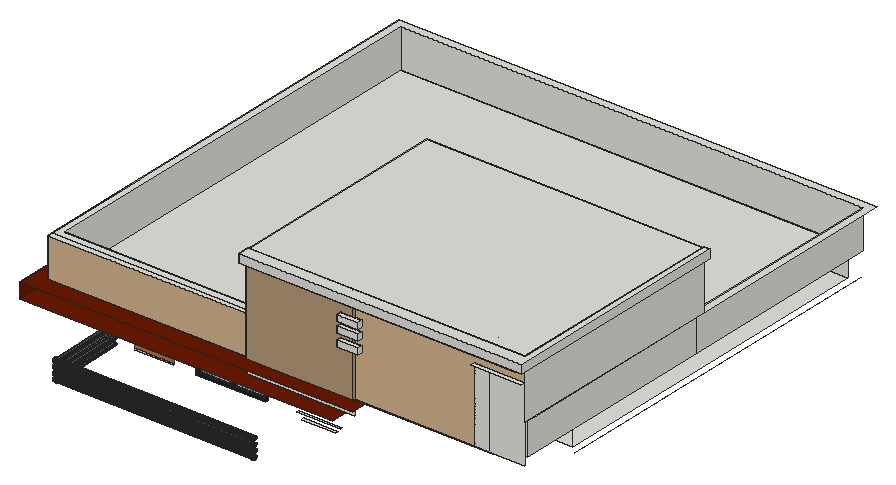
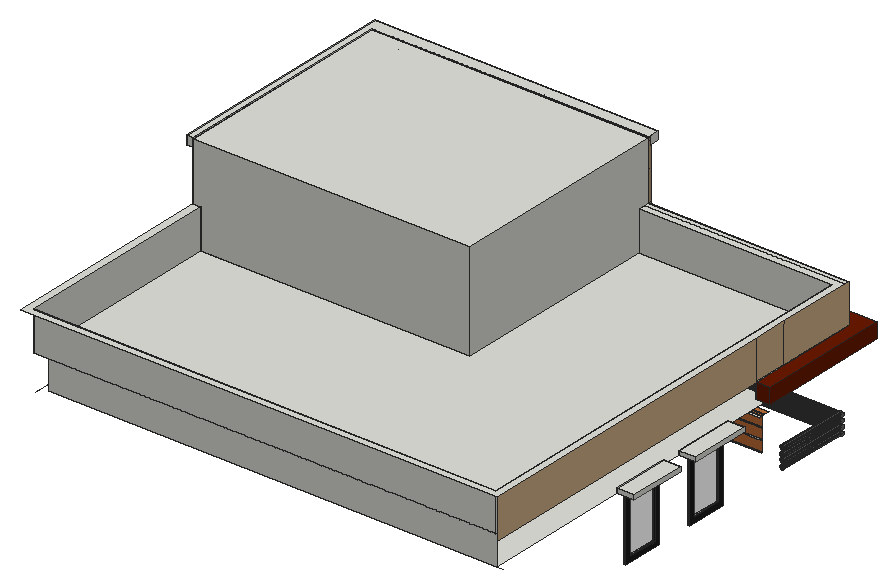
# SketchUp Ruby script. Lengths in inches.
U = 1.inch
M = Sketchup.active_model
def pt(a) = Geom::Point3d.new(a.map { |v| v * U })
def face(e, loops, mat)
  f = e.add_face(loops[0].map { |a| pt(a) })
  loops[1..].each { |l| e.add_face(l.map { |a| pt(a) }).erase! }
  f.material = f.back_material = mat if mat
  f
end
# faces: each face lists its corners as indices into pts; further lists are holes
def faces(e, pts, list, mat = nil) = list.each { |f| face(e, (f[0].is_a?(Array) ? f : [f]).map { |l| l.map { |i| pts[i] } }, mat) }
# xy, xz, yz: faces in a plane at the given z, y or x. An outline is a flat list of corners, or four numbers for a rectangle; further outlines are holes
def ring(l) = l.size == 4 ? [[l[0], l[1]], [l[2], l[1]], [l[2], l[3]], [l[0], l[3]]] : l.each_slice(2).to_a
def flat(e, list, mat, &to3) = list.each { |f| face(e, (f[0].is_a?(Array) ? f : [f]).map { |l| ring(l).map { |u, v| to3.(u, v) } }, mat) }
def xy(e, z, list, mat = nil) = flat(e, list, mat) { |x, y| [x, y, z] }
def xz(e, y, list, mat = nil) = flat(e, list, mat) { |x, z| [x, y, z] }
def yz(e, x, list, mat = nil) = flat(e, list, mat) { |y, z| [x, y, z] }
def lines(e, pts, list) = list.each { |a, b| e.add_line(pt(pts[a]), pt(pts[b])) }
# prism: a flat outline (further loops are holes) pulled along v
def prism(e, loops, v, mat = nil)
  f = face(e, loops, mat); d = Geom::Vector3d.new(v.map { |x| x * U })
  f.pushpull(f.normal.samedirection?(d) ? d.length : -d.length)
end
def box(e, o, s, mat = nil) = prism(e, [[o, [o[0] + s[0], o[1], o[2]], [o[0] + s[0], o[1] + s[1], o[2]], [o[0], o[1] + s[1], o[2]]]], [0, 0, s[2]], mat)
def at(x, y, z, deg = 0) = Geom::Transformation.translation(pt([x, y, z])) * Geom::Transformation.rotation(ORIGIN, Z_AXIS, deg.degrees)
def axes(o, x, y, z) = Geom::Transformation.new([*x, 0, *y, 0, *z, 0, *pt(o).to_a, 1])
def part(name) = M.definitions.add(name)
# library, detail: a bought-in or finely detailed component or shape, given as its bounding box
def library(name, o, s) = part(name).tap { |d| box(d.entities, o, s) }
def detail(e, o, s) = box(e.add_group.entities, o, s)
def put(e, d, t, mat = nil) = e.add_instance(d, t).tap { |i| i.material = mat if mat }
def group(e, t, mat = nil) = e.add_group.tap { |g| g.transformation = t; g.material = mat if mat }.entities
root = M.entities
M.materials.add("[0035_Tan]").color = [181, 154, 120]
M.materials.add("[0035_Tan]1").color = [210, 180, 140]
M.materials.add("[0134_DimGray]").color = [105, 105, 105]
M.materials.add("[Color B07]").color = [107, 26, 0]
M.materials.add("[Color M08]").color = [30, 30, 30]
M.materials.add("[Translucent Glass Blue]").color = [61, 91, 145]
M.materials["[Translucent Glass Blue]"].alpha = 0.5
M.materials.add("[Translucent Glass Gray]").color = [128, 128, 128]
M.materials["[Translucent Glass Gray]"].alpha = 0.5
M.materials.add("[Wood Veneer 01]").color = [191, 111, 58]
prism(root,[[[13.875,208.16,859.6875],[13.875,283.03,859.6875],[34.875,283.03,859.6875],[34.875,273.28,859.6875],[34.875,208.16,859.6875]]],[0,0,5.375])
prism(root,[[[34.875,378.1,859.6875],[34.875,312.97,859.6875],[34.875,306.78,859.6875],[13.875,306.78,859.6875],[13.875,378.1,859.6875]]],[0,0,5.375])
xy(root,777.125,[[141.33,116.9375,227.02,119.9375]])
xy(root,777.36,[[31.875,219.0625,34.875,270.0625]])
xy(root,777.36,[[31.875,317.1875,34.875,368.1875]],"[Color M08]")
xy(root,780.125,[[144.33,116.9375,184.18,119.9375],[187.18,116.9375,224.02,119.9375]],"[Color M08]")
xy(root,783.36,[[31.875,225.0625,34.875,264.0625],[31.875,323.1875,34.875,362.1875]],"[Color M08]")
xy(root,819,[[65.96,116.9375,113.96,119.9375]])
xy(root,819,[[65.96,113.9375,113.96,116.9375]],"[Wood Veneer 01]")
xy(root,825,[[59.96,113.9375,119.96,119.9375]],"[Wood Veneer 01]")
xy(root,834.8125,[[144.33,116.9375,184.18,119.9375],[187.18,116.9375,224.02,119.9375]],"[Color M08]")
xy(root,837.8125,[[141.33,116.9375,227.02,119.9375]],"[Color M08]")
xy(root,844.6875,[[350.38,17.9375,392.07,20.9375]])
xy(root,850.6875,[[344.38,17.9375,398.07,20.9375]])
xy(root,851.18,[[31.875,225.0625,34.875,264.0625],[31.875,323.1875,34.875,362.1875]],"[Color M08]")
xy(root,852,[[43.875,128.9375,595.125,552.98]])
xy(root,857.18,[[31.875,219.0625,34.875,270.0625],[31.875,317.1875,34.875,368.1875]],"[Color M08]")
xy(root,869.45,[[18.22,0,18.22,164.4375,35.6,164.4375,35.6,26.9375,282.125,26.9375,282.125,20.9375,402.53,20.9375,402.53,0]],"[Color B07]")
xy(root,882.89,[[35.6,26.9375,35.6,119.9375,578.6875,119.9375,578.6875,35.9375,282.125,35.9375,282.125,26.9375],[282.125,26.9375,578.6875,35.9375]])
xy(root,888,[[282.125,17.9375,413.18,20.9375],[35.6,20.9375,578.6875,26.9375],[44.6,35.9375,282.125,35.9375,282.125,296,614,296,614,552.98,44.6,552.98],[282.125,35.9375,614,296],[34.875,119.9375,35.6,128.9375],
  [34.875,128.9375,35.6,164.4375]])
xy(root,888,[[18.22,0,427.625,0,427.625,20.9375,413.18,20.9375,413.18,17.9375,282.125,17.9375,282.125,20.9375,35.6,20.9375,35.6,119.9375,34.875,119.9375,34.875,164.4375,18.22,164.4375]],"[Color B07]")
xy(root,936,[[35.6,20.9375,282.125,26.9375],[35.6,26.9375,282.125,26.9375,282.125,35.9375,44.6,35.9375,44.6,552.98,614,552.98,614,296,623,296,623,561.98,34.875,561.98,34.875,164.4375,35.6,164.4375],[282.125,26.9375,578.6875,35.9375],[578.6875,26.9375,623,35.9375],[614,35.9375,623,296]])
xy(root,944.65,[[398.24,11.9375,424.12,17.9375]])
xy(root,952.1,[[398.24,11.9375,424.12,17.9375]])
xy(root,959.84,[[398.24,11.9375,424.12,17.9375]])
xy(root,967.29,[[398.24,11.9375,424.12,17.9375]])
xy(root,972.59,[[398.24,11.9375,424.12,17.9375]])
xy(root,980,[[561.08,14.9375,623,20.9375]])
xy(root,980.04,[[398.24,11.9375,424.12,17.9375]])
xy(root,998.73,[[282.125,5.9375,282.125,17.9375,413.18,17.9375,413.18,20.9375,623,20.9375,623,5.9375],[623,5.9375,630.81,296]])
xy(root,1008,[[282.125,20.9375,623,296]])
xy(root,1009.125,[[282.125,5.9375,630.81,5.9375,630.81,296,623,296,623,20.9375,282.125,20.9375]])
xz(root,5.9375,[[282.125,998.73,630.81,1009.125]])
xz(root,11.9375,[[398.24,944.65,424.12,952.1],[398.24,959.84,424.12,967.29],[398.24,972.59,424.12,980.04]])
xz(root,17.9375,[[398.24,944.65,413.18,952.1],[413.18,944.65,424.12,952.1],[398.24,959.84,413.18,967.29],[413.18,959.84,424.12,967.29],[398.24,972.59,413.18,980.04],
  [413.18,972.59,424.12,980.04]])
xz(root,17.9375,[[282.125,888,413.18,888,413.18,944.65,398.24,944.65,398.24,952.1,413.18,952.1,413.18,959.84,398.24,959.84,398.24,967.29,413.18,967.29,413.18,972.59,398.24,972.59,398.24,980.04,413.18,980.04,413.18,998.73,282.125,998.73]],"[0035_Tan]")
xz(root,20.9375,[[282.125,869.45,413.18,888],[282.125,888,413.18,1008],[561.08,888,578.6875,980],[578.6875,888,623,980],[413.18,998.73,623,1008],
  [282.125,1008,623,1009.125]])
xz(root,20.9375,[[35.6,888,282.125,936],[413.18,888,561.08,888,561.08,980,623,980,623,998.73,413.18,998.73]],"[0035_Tan]1")
xz(root,26.9375,[[35.6,882.89,578.6875,888]])
xz(root,26.9375,[[35.6,869.45,282.125,882.89]],"[Color B07]")
xz(root,35.9375,[[44.6,888,282.125,936],[282.125,888,578.6875,936],[578.6875,888,614,936]])
xz(root,116.9375,[[65.96,778.55,113.96,779.87],[65.96,792.23,113.96,793.55],[65.96,805.92,113.96,807.24]])
xz(root,116.9375,[[[141.33,777.125,227.02,837.8125],[144.33,780.125,184.18,834.8125],[187.18,780.125,224.02,834.8125]]],"[Color M08]")
xz(root,116.9375,[[65.96,779.87,113.96,792.23],[65.96,793.55,113.96,805.92],[65.96,807.24,113.96,819]],"[Wood Veneer 01]")
xz(root,119.9375,[[[141.33,777.125,227.02,837.8125],[144.33,780.125,184.18,834.8125],[187.18,780.125,224.02,834.8125]],[34.875,852,35.6,882.89],[34.875,882.89,35.6,888]])
xz(root,119.9375,[[144.33,780.125,184.18,834.8125],[187.18,780.125,224.02,834.8125]],"[Translucent Glass Blue]")
xz(root,164.4375,[[34.875,888,35.6,936]])
xz(root,164.4375,[[18.22,869.45,35.6,888]],"[Color B07]")
xz(root,219.0625,[[31.875,777.36,34.875,857.18]],"[Color M08]")
xz(root,225.0625,[[31.875,783.36,34.875,851.18]],"[Color M08]")
xz(root,264.0625,[[31.875,783.36,34.875,851.18]],"[Color M08]")
xz(root,270.0625,[[31.875,777.36,34.875,857.18]],"[Color M08]")
xz(root,296,[[282.125,888,282.125,1008,623,1008,623,936,614,936,614,888],[623,998.73,630.81,1009.125]])
xz(root,317.1875,[[31.875,777.36,34.875,857.18]],"[Color M08]")
xz(root,323.1875,[[31.875,783.36,34.875,851.18]],"[Color M08]")
xz(root,362.1875,[[31.875,783.36,34.875,851.18]],"[Color M08]")
xz(root,368.1875,[[31.875,777.36,34.875,857.18]],"[Color M08]")
xz(root,552.98,[[43.875,852,595.125,888],[44.6,888,614,936]])
yz(root,18.22,[[0,869.45,164.4375,888]],"[Color B07]")
yz(root,31.875,[[[219.0625,777.36,270.0625,857.18],[225.0625,783.36,264.0625,851.18]],[[317.1875,777.36,368.1875,857.18],[323.1875,783.36,362.1875,851.18]]],"[Color M08]")
yz(root,34.875,[[[219.0625,777.36,270.0625,857.18],[225.0625,783.36,264.0625,851.18]],[[317.1875,777.36,368.1875,857.18],[323.1875,783.36,362.1875,851.18]]])
yz(root,34.875,[[164.4375,888,561.98,936]],"[0035_Tan]1")
yz(root,34.875,[[31.46,770.43,30.85,770.51,30.27,770.75,29.78,771.125,29.4,771.62,29.17,772.19,29.09,772.81,29.17,773.42,29.4,773.99,29.78,774.48,30.27,774.86,30.85,775.1,31.46,775.18,32.08,775.1,32.65,774.86,33.14,774.48,33.52,773.99,33.76,773.42,33.84,772.81,33.76,772.19,33.52,771.62,33.14,771.125,32.65,770.75,32.08,770.51],[31.46,777.49,30.85,777.57,30.27,777.8125,29.78,778.1875,29.4,778.68,29.17,779.25,29.09,779.87,29.17,780.48,29.4,781.06,29.78,781.55,30.27,781.92,30.85,782.16,31.46,782.24,32.08,782.16,32.65,781.92,33.14,781.55,33.52,781.06,33.76,780.48,33.84,779.87,33.76,779.25,33.52,778.68,33.14,778.1875,32.65,777.8125,32.08,777.57],[31.46,784.56,30.85,784.64,30.27,784.875,29.78,785.25,29.4,785.74,29.17,786.32,29.09,786.93,29.17,787.54,29.4,788.12,29.78,788.61,30.27,788.99,30.85,789.22,31.46,789.31,32.08,789.22,32.65,788.99,33.14,788.61,33.52,788.12,33.76,787.54,33.84,786.93,33.76,786.32,33.52,785.74,33.14,785.25,32.65,784.875,32.08,784.64],[31.46,791.62,30.85,791.7,30.27,791.9375,29.78,792.3125,29.4,792.81,29.17,793.38,29.09,793.99,29.17,794.61,29.4,795.18,29.78,795.67,30.27,796.05,30.85,796.29,31.46,796.37,32.08,796.29,32.65,796.05,33.14,795.67,33.52,795.18,33.76,794.61,33.84,793.99,33.76,793.38,33.52,792.81,33.14,792.3125,32.65,791.9375,32.08,791.7]],"[0134_DimGray]")
yz(root,34.875,[[225.0625,783.36,264.0625,851.18],[323.1875,783.36,362.1875,851.18]],"[Translucent Glass Gray]")
yz(root,35.6,[[119.9375,869.45,164.4375,882.89],[26.9375,882.89,119.9375,888],[119.9375,882.89,164.4375,888]])
yz(root,35.6,[[20.9375,888,119.9375,936],[119.9375,888,164.4375,936]],"[0035_Tan]1")
yz(root,35.6,[[26.9375,869.45,119.9375,882.89]],"[Color B07]")
yz(root,44.6,[[35.9375,888,552.98,936]])
yz(root,141.33,[[116.9375,777.125,119.9375,837.8125]],"[Color M08]")
yz(root,144.33,[[116.9375,780.125,119.9375,834.8125]],"[Color M08]")
yz(root,184.18,[[116.9375,780.125,119.9375,834.8125]],"[Color M08]")
yz(root,187.18,[[116.9375,780.125,119.9375,834.8125]],"[Color M08]")
yz(root,224.02,[[116.9375,780.125,119.9375,834.8125]],"[Color M08]")
yz(root,227.02,[[116.9375,777.125,119.9375,837.8125]],"[Color M08]")
yz(root,282.125,[[26.9375,869.45,35.9375,882.89],[35.9375,888,35.9375,936,20.9375,936,20.9375,1008,296,1008,296,888],[5.9375,998.73,17.9375,1009.125]])
yz(root,282.125,[[17.9375,888,20.9375,936],[17.9375,936,20.9375,1009.125]],"[0035_Tan]")
yz(root,398.24,[[11.9375,944.65,17.9375,952.1],[11.9375,959.84,17.9375,967.29],[11.9375,972.59,17.9375,980.04]])
yz(root,413.18,[[17.9375,888,20.9375,998.73]],"[0035_Tan]")
yz(root,424.12,[[11.9375,944.65,17.9375,952.1],[11.9375,959.84,17.9375,967.29],[11.9375,972.59,17.9375,980.04]])
yz(root,614,[[35.9375,888,296,936],[296,888,552.98,936]])
yz(root,623,[[20.9375,936,296,998.73],[20.9375,998.73,296,1008],[20.9375,1008,296,1009.125]])
yz(root,630.81,[[5.9375,998.73,296,1009.125]])
p = [[37.62,119.9375,771.45],[38.23,119.9375,771.37],[38.55,30.27,770.18],[37.9375,30.27,770.26],[38.85,119.9375,771.45],[39.17,30.27,770.26],
  [37.04,119.9375,771.69],[37.36,30.27,770.5],[39.42,119.9375,771.69],[39.74,30.27,770.5],[282.125,31.46,770.43],[282.125,30.85,770.51],
  [34.875,30.85,770.51],[34.875,31.46,770.43],[282.125,32.08,770.51],[34.875,32.08,770.51],[282.125,30.27,770.75],[40.0625,30.27,770.75],
  [37.04,30.27,770.75],[34.875,30.27,770.75],[36.55,119.9375,772.07],[36.87,30.27,770.875],[39.91,119.9375,772.07],[40.23,30.27,770.875],
  [282.125,32.65,770.75],[34.875,32.65,770.75],[282.125,29.78,771.125],[34.875,29.78,771.125],[282.125,33.14,771.125],[34.875,33.14,771.125],
  [36.49,30.27,771.37],[36.18,119.9375,772.56],[40.29,119.9375,772.56],[40.61,30.27,771.37],[282.125,29.4,771.62],[34.875,29.4,771.62],
  [282.125,33.52,771.62],[34.875,33.52,771.62],[36.26,30.27,771.94],[35.9375,119.9375,773.13],[40.53,119.9375,773.13],[40.85,30.27,771.94],
  [282.125,29.17,772.19],[34.875,29.17,772.19],[282.125,33.76,772.19],[34.875,33.76,772.19],[36.18,30.27,772.56],[35.86,119.9375,773.75],
  [36.22,30.27,772.24],[40.61,119.9375,773.75],[40.93,30.27,772.56],[40.88,30.27,772.24],[282.125,29.09,772.81],[34.875,29.09,772.81],
  [282.125,33.84,772.81],[34.875,33.84,772.81],[36.26,30.27,773.17],[35.9375,119.9375,774.36],[40.53,119.9375,774.36],[40.85,30.27,773.17],
  [282.125,29.17,773.42],[34.875,29.17,773.42],[282.125,33.76,773.42],[34.875,33.76,773.42],[36.49,30.27,773.74],[36.18,119.9375,774.94],
  [40.29,119.9375,774.94],[40.61,30.27,773.74],[282.125,29.4,773.99],[34.875,29.4,773.99],[282.125,33.52,773.99],[34.875,33.52,773.99],
  [36.87,30.27,774.23],[36.55,119.9375,775.43],[39.91,119.9375,775.43],[40.23,30.27,774.23],[282.125,29.78,774.48],[34.875,29.78,774.48],
  [282.125,33.14,774.48],[34.875,33.14,774.48],[37.36,30.27,774.61],[37.04,119.9375,775.8],[39.42,119.9375,775.8],[39.74,30.27,774.61],
  [282.125,30.27,774.86],[39.07,30.27,774.86],[38.03,30.27,774.86],[34.875,30.27,774.86],[282.125,32.65,774.86],[34.875,32.65,774.86],
  [37.9375,30.27,774.85],[37.62,119.9375,776.04],[38.85,119.9375,776.04],[39.17,30.27,774.85],[38.55,30.27,774.93],[38.23,119.9375,776.12],
  [282.125,30.85,775.1],[34.875,30.85,775.1],[282.125,32.08,775.1],[34.875,32.08,775.1],[282.125,31.46,775.18],[34.875,31.46,775.18],
  [282.125,31.46,777.49],[282.125,30.85,777.57],[34.875,30.85,777.57],[34.875,31.46,777.49],[282.125,32.08,777.57],[34.875,32.08,777.57],
  [282.125,30.27,777.8125],[39.59,30.27,777.8125],[37.51,30.27,777.8125],[34.875,30.27,777.8125],[37.04,119.9375,779.07],[37.62,119.9375,778.83],
  [37.9375,30.27,777.64],[37.36,30.27,777.875],[38.23,119.9375,778.75],[38.55,30.27,777.56],[38.85,119.9375,778.83],[39.17,30.27,777.64],
  [39.42,119.9375,779.07],[39.74,30.27,777.875],[282.125,32.65,777.8125],[34.875,32.65,777.8125],[282.125,29.78,778.1875],[34.875,29.78,778.1875],
  [282.125,33.14,778.1875],[34.875,33.14,778.1875],[36.55,119.9375,779.44],[37.04,30.27,778.125],[36.87,30.27,778.25],[39.91,119.9375,779.44],
  [40.23,30.27,778.25],[40.0625,30.27,778.125],[282.125,29.4,778.68],[34.875,29.4,778.68],[282.125,33.52,778.68],[34.875,33.52,778.68],
  [36.49,30.27,778.74],[36.18,119.9375,779.94],[40.29,119.9375,779.94],[40.61,30.27,778.74],[282.125,29.17,779.25],[34.875,29.17,779.25],
  [36.26,30.27,779.32],[35.9375,119.9375,780.51],[40.53,119.9375,780.51],[40.85,30.27,779.32],[282.125,33.76,779.25],[34.875,33.76,779.25],
  [282.125,29.09,779.87],[34.875,29.09,779.87],[36.18,30.27,779.93],[35.86,119.9375,781.12],[36.22,30.27,779.61],[40.61,119.9375,781.12],
  [40.93,30.27,779.93],[40.88,30.27,779.61],[282.125,33.84,779.87],[34.875,33.84,779.87],[282.125,29.17,780.48],[34.875,29.17,780.48],
  [36.26,30.27,780.54],[35.9375,119.9375,781.74],[40.53,119.9375,781.74],[40.85,30.27,780.54],[282.125,33.76,780.48],[34.875,33.76,780.48],
  [282.125,29.4,781.06],[34.875,29.4,781.06],[36.49,30.27,781.12],[36.18,119.9375,782.31],[40.29,119.9375,782.31],[40.61,30.27,781.12],
  [282.125,33.52,781.06],[34.875,33.52,781.06],[282.125,29.78,781.55],[34.875,29.78,781.55],[36.87,30.27,781.61],[36.55,119.9375,782.8],
  [39.91,119.9375,782.8],[40.23,30.27,781.61],[282.125,33.14,781.55],[34.875,33.14,781.55],[282.125,30.27,781.92],[39.82,30.27,781.92],
  [37.28,30.27,781.92],[34.875,30.27,781.92],[282.125,32.65,781.92],[34.875,32.65,781.92],[37.36,30.27,781.99],[37.04,119.9375,783.18],
  [39.42,119.9375,783.18],[39.74,30.27,781.99],[282.125,30.85,782.16],[34.875,30.85,782.16],[282.125,32.08,782.16],[34.875,32.08,782.16],
  [37.9375,30.27,782.22],[37.62,119.9375,783.42],[38.85,119.9375,783.42],[39.17,30.27,782.22],[38.03,30.27,782.24],[38.55,30.27,782.31],
  [38.23,119.9375,783.5],[39.07,30.27,782.24],[282.125,31.46,782.24],[34.875,31.46,782.24],[37.62,119.9375,785.39],[38.23,119.9375,785.31],
  [38.55,30.27,784.12],[37.9375,30.27,784.2],[38.85,119.9375,785.39],[39.17,30.27,784.2],[37.04,119.9375,785.63],[37.51,30.27,784.375],
  [37.36,30.27,784.4375],[39.42,119.9375,785.63],[39.74,30.27,784.4375],[39.59,30.27,784.375],[36.55,119.9375,786.01],[37.04,30.27,784.6875],
  [36.87,30.27,784.8125],[39.91,119.9375,786.01],[40.23,30.27,784.8125],[40.0625,30.27,784.6875],[282.125,30.85,784.64],[282.125,30.27,784.875],
  [40.28,30.27,784.875],[36.83,30.27,784.875],[34.875,30.27,784.875],[34.875,30.85,784.64],[282.125,31.46,784.56],[34.875,31.46,784.56],
  [282.125,32.08,784.64],[34.875,32.08,784.64],[282.125,32.65,784.875],[34.875,32.65,784.875],[36.49,30.27,785.31],[36.18,119.9375,786.5],
  [40.29,119.9375,786.5],[40.61,30.27,785.31],[282.125,29.78,785.25],[34.875,29.78,785.25],[282.125,33.14,785.25],[34.875,33.14,785.25],
  [282.125,29.4,785.74],[34.875,29.4,785.74],[36.26,30.27,785.88],[35.9375,119.9375,787.07],[40.53,119.9375,787.07],[40.85,30.27,785.88],
  [282.125,33.52,785.74],[34.875,33.52,785.74],[282.125,29.17,786.32],[34.875,29.17,786.32],[282.125,33.76,786.32],[34.875,33.76,786.32],
  [36.18,30.27,786.49],[35.86,119.9375,787.69],[36.22,30.27,786.18],[40.61,119.9375,787.69],[40.93,30.27,786.49],[40.88,30.27,786.18],
  [282.125,29.09,786.93],[34.875,29.09,786.93],[282.125,33.84,786.93],[34.875,33.84,786.93],[36.26,30.27,787.11],[35.9375,119.9375,788.3],
  [40.53,119.9375,788.3],[40.85,30.27,787.11],[282.125,29.17,787.54],[34.875,29.17,787.54],[282.125,33.76,787.54],[34.875,33.76,787.54],
  [36.49,30.27,787.68],[36.18,119.9375,788.87],[40.29,119.9375,788.87],[40.61,30.27,787.68],[282.125,29.4,788.12],[34.875,29.4,788.12],
  [282.125,33.52,788.12],[34.875,33.52,788.12],[36.87,30.27,788.17],[36.55,119.9375,789.36],[39.91,119.9375,789.36],[40.23,30.27,788.17],
  [282.125,29.78,788.61],[34.875,29.78,788.61],[282.125,33.14,788.61],[34.875,33.14,788.61],[37.28,30.27,788.49],[37.36,30.27,788.55],
  [37.04,119.9375,789.74],[39.42,119.9375,789.74],[39.74,30.27,788.55],[39.82,30.27,788.49],[37.9375,30.27,788.79],[37.62,119.9375,789.98],
  [38.85,119.9375,789.98],[39.17,30.27,788.79],[282.125,30.27,788.99],[34.875,30.27,788.99],[282.125,32.65,788.99],[34.875,32.65,788.99],
  [38.03,30.27,788.8],[38.55,30.27,788.87],[38.23,119.9375,790.06],[39.07,30.27,788.8],[282.125,30.85,789.22],[34.875,30.85,789.22],
  [282.125,32.08,789.22],[34.875,32.08,789.22],[282.125,31.46,789.31],[34.875,31.46,789.31],[282.125,31.46,791.62],[282.125,30.85,791.7],
  [34.875,30.85,791.7],[34.875,31.46,791.62],[282.125,32.08,791.7],[34.875,32.08,791.7],[282.125,30.27,791.9375],[38.59,30.27,791.9375],
  [38.51,30.27,791.9375],[34.875,30.27,791.9375],[282.125,32.65,791.9375],[34.875,32.65,791.9375],[282.125,29.78,792.3125],[34.875,29.78,792.3125],
  [37.62,119.9375,793.2],[38.23,119.9375,793.12],[38.55,30.27,791.93],[37.9375,30.27,792.01],[38.85,119.9375,793.2],[39.17,30.27,792.01],
  [282.125,33.14,792.3125],[34.875,33.14,792.3125],[37.04,119.9375,793.44],[37.51,30.27,792.1875],[37.36,30.27,792.25],[39.42,119.9375,793.44],
  [39.74,30.27,792.25],[39.59,30.27,792.1875],[36.55,119.9375,793.82],[37.04,30.27,792.5],[36.87,30.27,792.625],[39.91,119.9375,793.82],
  [40.23,30.27,792.625],[40.0625,30.27,792.5],[282.125,29.4,792.81],[34.875,29.4,792.81],[282.125,33.52,792.81],[34.875,33.52,792.81],
  [36.49,30.27,793.12],[36.18,119.9375,794.31],[36.83,30.27,792.6875],[40.29,119.9375,794.31],[40.61,30.27,793.12],[40.28,30.27,792.6875],
  [282.125,29.17,793.38],[34.875,29.17,793.38],[282.125,33.76,793.38],[34.875,33.76,793.38],[36.26,30.27,793.69],[35.9375,119.9375,794.88],
  [40.53,119.9375,794.88],[40.85,30.27,793.69],[282.125,29.09,793.99],[34.875,29.09,793.99],[282.125,33.84,793.99],[34.875,33.84,793.99],
  [36.18,30.27,794.31],[35.86,119.9375,795.5],[36.22,30.27,793.99],[40.61,119.9375,795.5],[40.93,30.27,794.31],[40.88,30.27,793.99],
  [282.125,29.17,794.61],[34.875,29.17,794.61],[282.125,33.76,794.61],[34.875,33.76,794.61],[36.26,30.27,794.92],[35.9375,119.9375,796.11],
  [40.53,119.9375,796.11],[40.85,30.27,794.92],[282.125,29.4,795.18],[34.875,29.4,795.18],[282.125,33.52,795.18],[34.875,33.52,795.18],
  [36.49,30.27,795.49],[36.18,119.9375,796.69],[40.29,119.9375,796.69],[40.61,30.27,795.49],[282.125,29.78,795.67],[34.875,29.78,795.67],
  [282.125,33.14,795.67],[34.875,33.14,795.67],[36.87,30.27,795.98],[36.55,119.9375,797.18],[39.91,119.9375,797.18],[40.23,30.27,795.98],
  [282.125,30.27,796.05],[40.15,30.27,796.05],[36.96,30.27,796.05],[34.875,30.27,796.05],[282.125,32.65,796.05],[34.875,32.65,796.05],
  [282.125,30.85,796.29],[34.875,30.85,796.29],[37.28,30.27,796.3],[37.36,30.27,796.36],[37.04,119.9375,797.55],[39.42,119.9375,797.55],
  [39.74,30.27,796.36],[39.82,30.27,796.3],[282.125,32.08,796.29],[34.875,32.08,796.29],[282.125,31.46,796.37],[34.875,31.46,796.37],
  [37.9375,30.27,796.6],[37.62,119.9375,797.79],[38.85,119.9375,797.79],[39.17,30.27,796.6],[38.03,30.27,796.61],[38.55,30.27,796.68],
  [38.23,119.9375,797.87],[39.07,30.27,796.61],[43.875,552.98,852],[35.6,552.98,852],[604.125,119.9375,852],[604.125,561.98,852],
  [595.125,128.9375,852],[595.125,128.9375,888],[578.6875,35.9375,936],[578.6875,35.9375,1008],[578.6875,26.9375,936],[578.6875,20.9375,936],
  [413.18,17.9375,1009.125],[413.18,17.9375,998.73]]
faces(root,p,[[0,1,2,3],[1,4,5,2],[6,0,3,7],[4,8,9,5],[10,11,12,13],[14,10,13,15],[11,16,17,18,19,12],[20,6,7,18,21],
  [8,22,23,17,9],[24,14,15,25],[16,26,27,19,18,17],[28,24,25,29],[30,31,20,21],[23,22,32,33],[26,34,35,27],[36,28,29,37],
  [38,39,31,30],[33,32,40,41],[34,42,43,35],[44,36,37,45],[46,47,39,38,48],[41,40,49,50,51],[42,52,53,43],[54,44,45,55],
  [56,57,47,46],[50,49,58,59],[52,60,61,53],[62,54,55,63],[64,65,57,56],[59,58,66,67],[60,68,69,61],[70,62,63,71],
  [72,73,65,64],[67,66,74,75],[68,76,77,69],[78,70,71,79],[73,72,80,81],[82,83,75,74],[76,84,85,86,87,77],[88,78,79,89],
  [81,80,90,91],[92,93,83,82],[91,90,86,94,95],[95,94,85,93,92],[84,96,97,87,86,85],[98,88,89,99],[96,100,101,97],[100,98,99,101],
  [102,103,104,105],[106,102,105,107],[103,108,109,110,111,104],[112,113,114,110,115],[113,116,117,114],[116,118,119,117],[118,120,121,109,119],[122,106,107,123],
  [108,124,125,111,110,109],[126,122,123,127],[128,112,115,129,130],[120,131,132,133,121],[124,134,135,125],[136,126,127,137],[138,139,128,130],[132,131,140,141],
  [134,142,143,135],[144,145,139,138],[141,140,146,147],[148,136,137,149],[142,150,151,143],[152,153,145,144,154],[147,146,155,156,157],[158,148,149,159],
  [150,160,161,151],[162,163,153,152],[156,155,164,165],[166,158,159,167],[160,168,169,161],[170,171,163,162],[165,164,172,173],[174,166,167,175],
  [168,176,177,169],[178,179,171,170],[173,172,180,181],[182,174,175,183],[176,184,185,186,187,177],[188,182,183,189],[179,178,186,190,191],[192,193,185,181,180],
  [184,194,195,187,186,185],[196,188,189,197],[191,190,198,199],[200,201,193,192],[199,198,202,203,204],[204,203,205,201,200],[194,206,207,195],[206,196,197,207],
  [208,209,210,211],[209,212,213,210],[214,208,211,215,216],[212,217,218,219,213],[220,214,216,221,222],[217,223,224,225,218],[226,227,228,229,230,231],[232,226,231,233],
  [234,232,233,235],[236,234,235,237],[238,239,220,222,229],[224,223,240,241,228],[227,242,243,230,229,228],[244,236,237,245],[242,246,247,243],[248,249,239,238],
  [241,240,250,251],[252,244,245,253],[246,254,255,247],[256,252,253,257],[258,259,249,248,260],[251,250,261,262,263],[254,264,265,255],[266,256,257,267],
  [268,269,259,258],[262,261,270,271],[264,272,273,265],[274,266,267,275],[276,277,269,268],[271,270,278,279],[272,280,281,273],[282,274,275,283],
  [284,285,277,276],[279,278,286,287],[280,288,289,281],[290,282,283,291],[285,284,292,293,294],[295,296,297,287,286],[294,293,298,299],[300,301,296,295],
  [288,302,303,289],[304,290,291,305],[299,298,306,307,308],[308,307,309,301,300],[302,310,311,303],[312,304,305,313],[310,314,315,311],[314,312,313,315],
  [316,317,318,319],[320,316,319,321],[317,322,323,324,325,318],[326,320,321,327],[322,328,329,325,324,323],[330,331,332,324,333],[331,334,335,323,332],[336,326,327,337],
  [338,330,333,339,340],[334,341,342,343,335],[344,338,340,345,346],[341,347,348,349,342],[328,350,351,329],[352,336,337,353],[354,355,344,346,356],[348,347,357,358,359],
  [350,360,361,351],[362,352,353,363],[364,365,355,354],[358,357,366,367],[360,368,369,361],[370,362,363,371],[372,373,365,364,374],[367,366,375,376,377],
  [368,378,379,369],[380,370,371,381],[382,383,373,372],[376,375,384,385],[378,386,387,379],[388,380,381,389],[390,391,383,382],[385,384,392,393],
  [386,394,395,387],[396,388,389,397],[398,399,391,390],[393,392,400,401],[394,402,403,404,405,395],[406,396,397,407],[402,408,409,405,404,403],[399,398,404,410,411,412],
  [413,414,415,403,401,400],[416,406,407,417],[408,418,419,409],[418,416,417,419],[412,411,420,421],[422,423,414,413],[421,420,424,425,426],[426,425,427,423,422]],"[0134_DimGray]")
lines(root,p,[[428,429],[430,431],[432,433],[434,435],[436,437],[438,439]])
